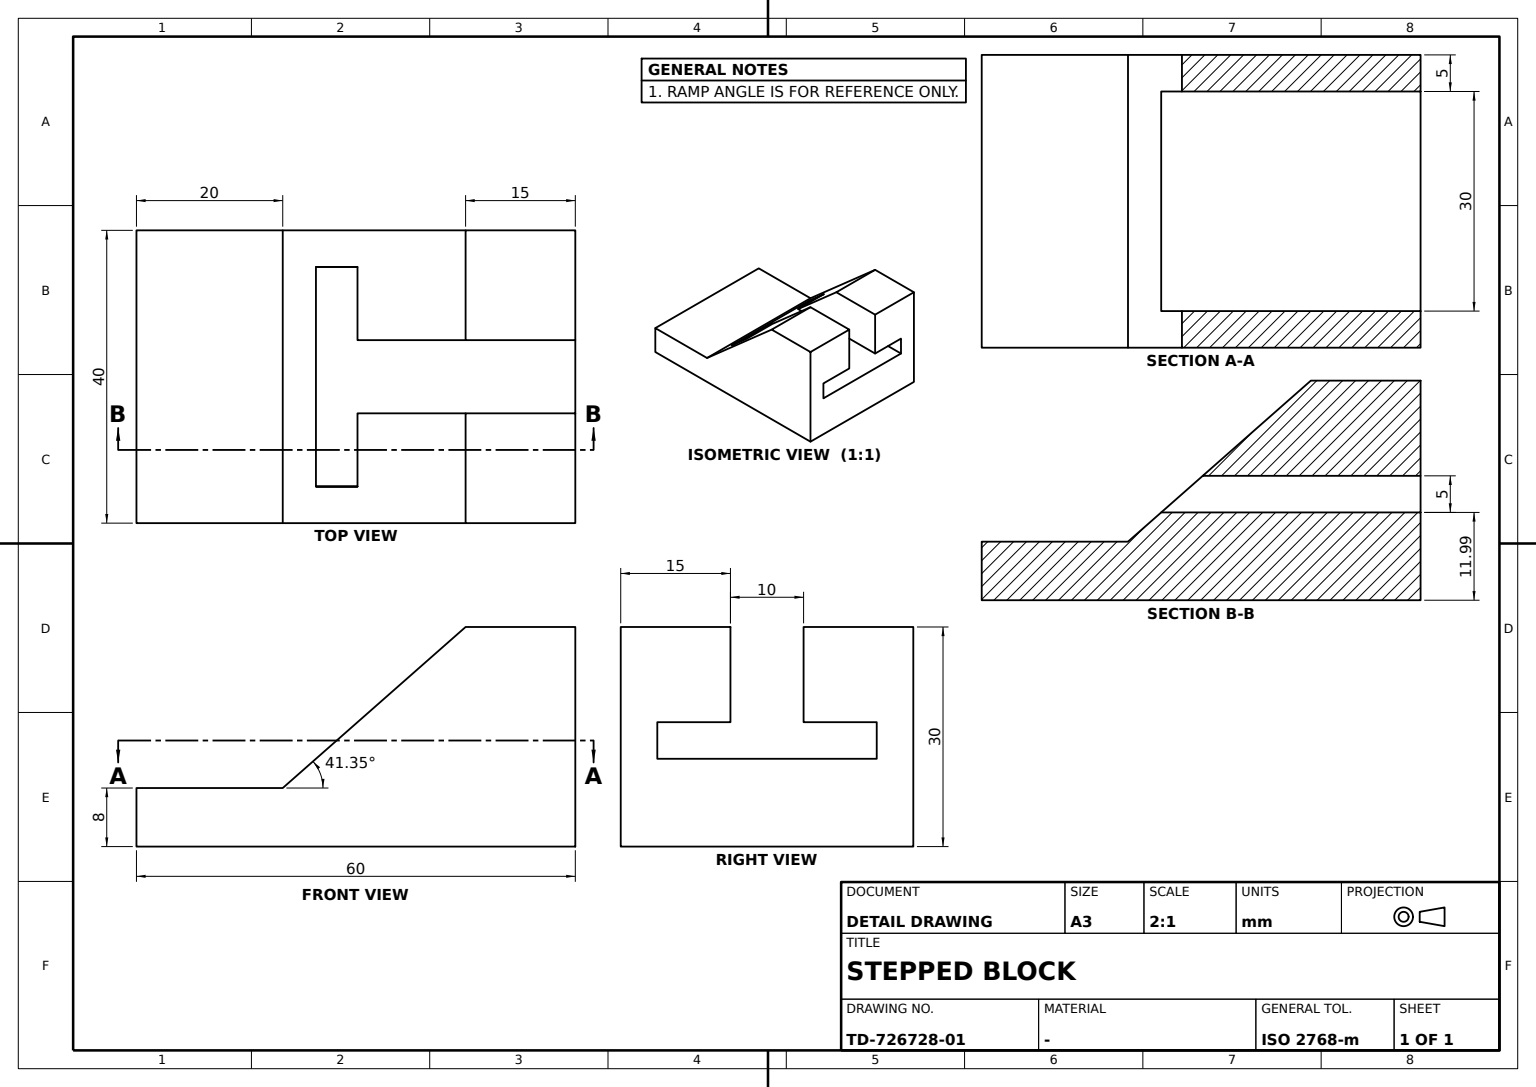
ISO-10303-21;
HEADER;
FILE_DESCRIPTION((''),'2;1');
FILE_NAME('','',(''),(''),'','','');
FILE_SCHEMA(('AUTOMOTIVE_DESIGN'));
ENDSEC;
DATA;
#1=APPLICATION_CONTEXT('');
#2=PRODUCT_CONTEXT('',#1,'mechanical');
#3=PRODUCT('','','',(#2));
#4=PRODUCT_DEFINITION_FORMATION('','',#3);
#5=PRODUCT_DEFINITION_CONTEXT('',#1,'design');
#6=PRODUCT_DEFINITION('','',#4,#5);
#7=PRODUCT_DEFINITION_SHAPE('','',#6);
#8=(LENGTH_UNIT()NAMED_UNIT(*)SI_UNIT(.MILLI.,.METRE.));
#9=(NAMED_UNIT(*)PLANE_ANGLE_UNIT()SI_UNIT($,.RADIAN.));
#10=(NAMED_UNIT(*)SI_UNIT($,.STERADIAN.)SOLID_ANGLE_UNIT());
#11=UNCERTAINTY_MEASURE_WITH_UNIT(LENGTH_MEASURE(0.005),#8,'distance_accuracy_value','');
#12=(GEOMETRIC_REPRESENTATION_CONTEXT(3)GLOBAL_UNCERTAINTY_ASSIGNED_CONTEXT((#11))GLOBAL_UNIT_ASSIGNED_CONTEXT((#8,#9,#10))REPRESENTATION_CONTEXT('',''));
#13=CARTESIAN_POINT('',(15.,-35.460872,11.994432));
#14=VERTEX_POINT('',#13);
#15=CARTESIAN_POINT('',(15.,-29.779054,16.994432));
#16=VERTEX_POINT('',#15);
#17=CARTESIAN_POINT('',(15.,-40.,8.));
#18=DIRECTION('',(0.,0.750713517,0.660627895));
#19=VECTOR('',#18,1000.);
#20=LINE('',#17,#19);
#21=EDGE_CURVE('',#14,#16,#20,.T.);
#22=ORIENTED_EDGE('',*,*,#21,.T.);
#23=CARTESIAN_POINT('',(15.,0.,16.994432));
#24=VERTEX_POINT('',#23);
#25=CARTESIAN_POINT('',(15.,-60.,16.994432));
#26=DIRECTION('',(0.,1.,0.));
#27=VECTOR('',#26,1000.);
#28=LINE('',#25,#27);
#29=EDGE_CURVE('',#16,#24,#28,.T.);
#30=ORIENTED_EDGE('',*,*,#29,.T.);
#31=CARTESIAN_POINT('',(15.,0.,11.994432));
#32=VERTEX_POINT('',#31);
#33=CARTESIAN_POINT('',(15.,0.,0.));
#34=DIRECTION('',(0.,0.,1.));
#35=VECTOR('',#34,1000.);
#36=LINE('',#33,#35);
#37=EDGE_CURVE('',#32,#24,#36,.T.);
#38=ORIENTED_EDGE('',*,*,#37,.F.);
#39=CARTESIAN_POINT('',(15.,-60.,11.994432));
#40=LINE('',#39,#27);
#41=EDGE_CURVE('',#14,#32,#40,.T.);
#42=ORIENTED_EDGE('',*,*,#41,.F.);
#43=EDGE_LOOP('',(#22,#30,#38,#42));
#44=FACE_BOUND('',#43,.T.);
#45=DIRECTION('',(-1.,0.,0.));
#46=AXIS2_PLACEMENT_3D('',#39,#45,#34);
#47=PLANE('',#46);
#48=ADVANCED_FACE('',(#44),#47,.T.);
#49=CARTESIAN_POINT('',(-20.,-60.,8.));
#50=VERTEX_POINT('',#49);
#51=CARTESIAN_POINT('',(-20.,-40.,8.));
#52=VERTEX_POINT('',#51);
#53=CARTESIAN_POINT('',(-20.,0.,8.));
#54=LINE('',#53,#27);
#55=EDGE_CURVE('',#50,#52,#54,.T.);
#56=ORIENTED_EDGE('',*,*,#55,.F.);
#57=CARTESIAN_POINT('',(20.,-60.,8.));
#58=VERTEX_POINT('',#57);
#59=CARTESIAN_POINT('',(0.,-60.,8.));
#60=DIRECTION('',(1.,0.,0.));
#61=VECTOR('',#60,1000.);
#62=LINE('',#59,#61);
#63=EDGE_CURVE('',#50,#58,#62,.T.);
#64=ORIENTED_EDGE('',*,*,#63,.T.);
#65=CARTESIAN_POINT('',(20.,-40.,8.));
#66=VERTEX_POINT('',#65);
#67=CARTESIAN_POINT('',(20.,0.,8.));
#68=LINE('',#67,#27);
#69=EDGE_CURVE('',#58,#66,#68,.T.);
#70=ORIENTED_EDGE('',*,*,#69,.T.);
#71=CARTESIAN_POINT('',(0.,-40.,8.));
#72=LINE('',#71,#61);
#73=EDGE_CURVE('',#52,#66,#72,.T.);
#74=ORIENTED_EDGE('',*,*,#73,.F.);
#75=EDGE_LOOP('',(#56,#64,#70,#74));
#76=FACE_BOUND('',#75,.T.);
#77=DIRECTION('',(0.,0.,-1.));
#78=AXIS2_PLACEMENT_3D('',#59,#77,#26);
#79=PLANE('',#78);
#80=ADVANCED_FACE('',(#76),#79,.F.);
#81=CARTESIAN_POINT('',(20.,0.,30.));
#82=VERTEX_POINT('',#81);
#83=CARTESIAN_POINT('',(20.,-15.,30.));
#84=VERTEX_POINT('',#83);
#85=DIRECTION('',(0.,-1.,0.));
#86=VECTOR('',#85,1000.);
#87=LINE('',#81,#86);
#88=EDGE_CURVE('',#82,#84,#87,.T.);
#89=ORIENTED_EDGE('',*,*,#88,.T.);
#90=CARTESIAN_POINT('',(20.,-21.424707,24.346258));
#91=LINE('',#90,#19);
#92=EDGE_CURVE('',#66,#84,#91,.T.);
#93=ORIENTED_EDGE('',*,*,#92,.F.);
#94=ORIENTED_EDGE('',*,*,#69,.F.);
#95=CARTESIAN_POINT('',(20.,-60.,0.));
#96=VERTEX_POINT('',#95);
#97=LINE('',#95,#35);
#98=EDGE_CURVE('',#96,#58,#97,.T.);
#99=ORIENTED_EDGE('',*,*,#98,.F.);
#100=CARTESIAN_POINT('',(20.,0.,0.));
#101=VERTEX_POINT('',#100);
#102=LINE('',#100,#86);
#103=EDGE_CURVE('',#101,#96,#102,.T.);
#104=ORIENTED_EDGE('',*,*,#103,.F.);
#105=LINE('',#100,#35);
#106=EDGE_CURVE('',#101,#82,#105,.T.);
#107=ORIENTED_EDGE('',*,*,#106,.T.);
#108=EDGE_LOOP('',(#89,#93,#94,#99,#104,#107));
#109=FACE_BOUND('',#108,.T.);
#110=AXIS2_PLACEMENT_3D('',#100,#60,#26);
#111=PLANE('',#110);
#112=ADVANCED_FACE('',(#109),#111,.T.);
#113=CARTESIAN_POINT('',(-5.,-29.779054,16.994432));
#114=VERTEX_POINT('',#113);
#115=CARTESIAN_POINT('',(-5.,0.,16.994432));
#116=VERTEX_POINT('',#115);
#117=CARTESIAN_POINT('',(-5.,-60.,16.994432));
#118=LINE('',#117,#27);
#119=EDGE_CURVE('',#114,#116,#118,.T.);
#120=ORIENTED_EDGE('',*,*,#119,.F.);
#121=CARTESIAN_POINT('',(-15.,-29.779054,16.994432));
#122=VERTEX_POINT('',#121);
#123=CARTESIAN_POINT('',(0.,-29.779054,16.994432));
#124=VECTOR('',#45,1000.);
#125=LINE('',#123,#124);
#126=EDGE_CURVE('',#114,#122,#125,.T.);
#127=ORIENTED_EDGE('',*,*,#126,.T.);
#128=CARTESIAN_POINT('',(-15.,0.,16.994432));
#129=VERTEX_POINT('',#128);
#130=CARTESIAN_POINT('',(-15.,-60.,16.994432));
#131=LINE('',#130,#27);
#132=EDGE_CURVE('',#122,#129,#131,.T.);
#133=ORIENTED_EDGE('',*,*,#132,.T.);
#134=CARTESIAN_POINT('',(0.,0.,16.994432));
#135=LINE('',#134,#124);
#136=EDGE_CURVE('',#116,#129,#135,.T.);
#137=ORIENTED_EDGE('',*,*,#136,.F.);
#138=EDGE_LOOP('',(#120,#127,#133,#137));
#139=FACE_BOUND('',#138,.T.);
#140=AXIS2_PLACEMENT_3D('',#25,#77,#45);
#141=PLANE('',#140);
#142=ADVANCED_FACE('',(#139),#141,.T.);
#143=CARTESIAN_POINT('',(5.,-29.779054,16.994432));
#144=VERTEX_POINT('',#143);
#145=CARTESIAN_POINT('',(5.,-15.,30.));
#146=VERTEX_POINT('',#145);
#147=CARTESIAN_POINT('',(5.,-40.,8.));
#148=LINE('',#147,#19);
#149=EDGE_CURVE('',#144,#146,#148,.T.);
#150=ORIENTED_EDGE('',*,*,#149,.F.);
#151=EDGE_CURVE('',#16,#144,#125,.T.);
#152=ORIENTED_EDGE('',*,*,#151,.F.);
#153=ORIENTED_EDGE('',*,*,#21,.F.);
#154=CARTESIAN_POINT('',(-15.,-35.460872,11.994432));
#155=VERTEX_POINT('',#154);
#156=CARTESIAN_POINT('',(0.,-35.460872,11.994432));
#157=LINE('',#156,#61);
#158=EDGE_CURVE('',#155,#14,#157,.T.);
#159=ORIENTED_EDGE('',*,*,#158,.F.);
#160=CARTESIAN_POINT('',(-15.,-40.,8.));
#161=DIRECTION('',(0.,-0.750713517,-0.660627895));
#162=VECTOR('',#161,1000.);
#163=LINE('',#160,#162);
#164=EDGE_CURVE('',#122,#155,#163,.T.);
#165=ORIENTED_EDGE('',*,*,#164,.F.);
#166=ORIENTED_EDGE('',*,*,#126,.F.);
#167=CARTESIAN_POINT('',(-5.,-15.,30.));
#168=VERTEX_POINT('',#167);
#169=CARTESIAN_POINT('',(-5.,-40.223483,7.803335));
#170=LINE('',#169,#19);
#171=EDGE_CURVE('',#114,#168,#170,.T.);
#172=ORIENTED_EDGE('',*,*,#171,.T.);
#173=CARTESIAN_POINT('',(-20.,-15.,30.));
#174=VERTEX_POINT('',#173);
#175=CARTESIAN_POINT('',(0.,-15.,30.));
#176=LINE('',#175,#61);
#177=EDGE_CURVE('',#174,#168,#176,.T.);
#178=ORIENTED_EDGE('',*,*,#177,.F.);
#179=CARTESIAN_POINT('',(-20.,-21.424707,24.346258));
#180=LINE('',#179,#19);
#181=EDGE_CURVE('',#52,#174,#180,.T.);
#182=ORIENTED_EDGE('',*,*,#181,.F.);
#183=ORIENTED_EDGE('',*,*,#73,.T.);
#184=ORIENTED_EDGE('',*,*,#92,.T.);
#185=EDGE_CURVE('',#146,#84,#176,.T.);
#186=ORIENTED_EDGE('',*,*,#185,.F.);
#187=EDGE_LOOP('',(#150,#152,#153,#159,#165,#166,#172,#178,#182,#183,#184,#186));
#188=FACE_BOUND('',#187,.T.);
#189=DIRECTION('',(0.,0.660627895,-0.750713517));
#190=AXIS2_PLACEMENT_3D('',#71,#189,#18);
#191=PLANE('',#190);
#192=ADVANCED_FACE('',(#188),#191,.F.);
#193=CARTESIAN_POINT('',(5.,0.,30.));
#194=VERTEX_POINT('',#193);
#195=LINE('',#193,#86);
#196=EDGE_CURVE('',#194,#146,#195,.T.);
#197=ORIENTED_EDGE('',*,*,#196,.F.);
#198=CARTESIAN_POINT('',(5.,0.,16.994432));
#199=VERTEX_POINT('',#198);
#200=CARTESIAN_POINT('',(5.,0.,0.));
#201=LINE('',#200,#35);
#202=EDGE_CURVE('',#199,#194,#201,.T.);
#203=ORIENTED_EDGE('',*,*,#202,.F.);
#204=CARTESIAN_POINT('',(5.,-60.,16.994432));
#205=LINE('',#204,#27);
#206=EDGE_CURVE('',#144,#199,#205,.T.);
#207=ORIENTED_EDGE('',*,*,#206,.F.);
#208=ORIENTED_EDGE('',*,*,#149,.T.);
#209=EDGE_LOOP('',(#197,#203,#207,#208));
#210=FACE_BOUND('',#209,.T.);
#211=AXIS2_PLACEMENT_3D('',#204,#45,#34);
#212=PLANE('',#211);
#213=ADVANCED_FACE('',(#210),#212,.T.);
#214=CARTESIAN_POINT('',(-5.,0.,30.));
#215=VERTEX_POINT('',#214);
#216=CARTESIAN_POINT('',(-5.,0.,30.276649));
#217=LINE('',#216,#35);
#218=EDGE_CURVE('',#116,#215,#217,.T.);
#219=ORIENTED_EDGE('',*,*,#218,.T.);
#220=CARTESIAN_POINT('',(-5.,-60.,30.));
#221=LINE('',#220,#86);
#222=EDGE_CURVE('',#215,#168,#221,.T.);
#223=ORIENTED_EDGE('',*,*,#222,.T.);
#224=ORIENTED_EDGE('',*,*,#171,.F.);
#225=ORIENTED_EDGE('',*,*,#119,.T.);
#226=EDGE_LOOP('',(#219,#223,#224,#225));
#227=FACE_BOUND('',#226,.T.);
#228=CARTESIAN_POINT('',(-5.,-60.,30.276649));
#229=AXIS2_PLACEMENT_3D('',#228,#60,#77);
#230=PLANE('',#229);
#231=ADVANCED_FACE('',(#227),#230,.T.);
#232=CARTESIAN_POINT('',(-20.,-60.,0.));
#233=VERTEX_POINT('',#232);
#234=CARTESIAN_POINT('',(0.,-60.,0.));
#235=LINE('',#234,#61);
#236=EDGE_CURVE('',#233,#96,#235,.T.);
#237=ORIENTED_EDGE('',*,*,#236,.F.);
#238=CARTESIAN_POINT('',(-20.,0.,0.));
#239=VERTEX_POINT('',#238);
#240=LINE('',#238,#86);
#241=EDGE_CURVE('',#239,#233,#240,.T.);
#242=ORIENTED_EDGE('',*,*,#241,.F.);
#243=CARTESIAN_POINT('',(0.,0.,0.));
#244=LINE('',#243,#61);
#245=EDGE_CURVE('',#239,#101,#244,.T.);
#246=ORIENTED_EDGE('',*,*,#245,.T.);
#247=ORIENTED_EDGE('',*,*,#103,.T.);
#248=EDGE_LOOP('',(#237,#242,#246,#247));
#249=FACE_BOUND('',#248,.T.);
#250=AXIS2_PLACEMENT_3D('',#243,#34,#85);
#251=PLANE('',#250);
#252=ADVANCED_FACE('',(#249),#251,.F.);
#253=CARTESIAN_POINT('',(-20.,0.,30.));
#254=VERTEX_POINT('',#253);
#255=LINE('',#253,#86);
#256=EDGE_CURVE('',#254,#174,#255,.T.);
#257=ORIENTED_EDGE('',*,*,#256,.T.);
#258=ORIENTED_EDGE('',*,*,#177,.T.);
#259=ORIENTED_EDGE('',*,*,#222,.F.);
#260=CARTESIAN_POINT('',(0.,0.,30.));
#261=LINE('',#260,#61);
#262=EDGE_CURVE('',#254,#215,#261,.T.);
#263=ORIENTED_EDGE('',*,*,#262,.F.);
#264=EDGE_LOOP('',(#257,#258,#259,#263));
#265=FACE_BOUND('',#264,.T.);
#266=AXIS2_PLACEMENT_3D('',#260,#34,#85);
#267=PLANE('',#266);
#268=ADVANCED_FACE('',(#265),#267,.T.);
#269=ORIENTED_EDGE('',*,*,#164,.T.);
#270=CARTESIAN_POINT('',(-15.,0.,11.994432));
#271=VERTEX_POINT('',#270);
#272=CARTESIAN_POINT('',(-15.,-60.,11.994432));
#273=LINE('',#272,#27);
#274=EDGE_CURVE('',#155,#271,#273,.T.);
#275=ORIENTED_EDGE('',*,*,#274,.T.);
#276=CARTESIAN_POINT('',(-15.,0.,0.));
#277=VECTOR('',#77,1000.);
#278=LINE('',#276,#277);
#279=EDGE_CURVE('',#129,#271,#278,.T.);
#280=ORIENTED_EDGE('',*,*,#279,.F.);
#281=ORIENTED_EDGE('',*,*,#132,.F.);
#282=EDGE_LOOP('',(#269,#275,#280,#281));
#283=FACE_BOUND('',#282,.T.);
#284=AXIS2_PLACEMENT_3D('',#130,#60,#77);
#285=PLANE('',#284);
#286=ADVANCED_FACE('',(#283),#285,.T.);
#287=EDGE_CURVE('',#24,#199,#135,.T.);
#288=ORIENTED_EDGE('',*,*,#287,.F.);
#289=ORIENTED_EDGE('',*,*,#29,.F.);
#290=ORIENTED_EDGE('',*,*,#151,.T.);
#291=ORIENTED_EDGE('',*,*,#206,.T.);
#292=EDGE_LOOP('',(#288,#289,#290,#291));
#293=FACE_BOUND('',#292,.T.);
#294=ADVANCED_FACE('',(#293),#141,.T.);
#295=ORIENTED_EDGE('',*,*,#158,.T.);
#296=ORIENTED_EDGE('',*,*,#41,.T.);
#297=CARTESIAN_POINT('',(0.,0.,11.994432));
#298=LINE('',#297,#61);
#299=EDGE_CURVE('',#271,#32,#298,.T.);
#300=ORIENTED_EDGE('',*,*,#299,.F.);
#301=ORIENTED_EDGE('',*,*,#274,.F.);
#302=EDGE_LOOP('',(#295,#296,#300,#301));
#303=FACE_BOUND('',#302,.T.);
#304=AXIS2_PLACEMENT_3D('',#272,#34,#60);
#305=PLANE('',#304);
#306=ADVANCED_FACE('',(#303),#305,.T.);
#307=ORIENTED_EDGE('',*,*,#299,.T.);
#308=ORIENTED_EDGE('',*,*,#37,.T.);
#309=ORIENTED_EDGE('',*,*,#287,.T.);
#310=ORIENTED_EDGE('',*,*,#202,.T.);
#311=EDGE_CURVE('',#194,#82,#261,.T.);
#312=ORIENTED_EDGE('',*,*,#311,.T.);
#313=ORIENTED_EDGE('',*,*,#106,.F.);
#314=ORIENTED_EDGE('',*,*,#245,.F.);
#315=LINE('',#238,#35);
#316=EDGE_CURVE('',#239,#254,#315,.T.);
#317=ORIENTED_EDGE('',*,*,#316,.T.);
#318=ORIENTED_EDGE('',*,*,#262,.T.);
#319=ORIENTED_EDGE('',*,*,#218,.F.);
#320=ORIENTED_EDGE('',*,*,#136,.T.);
#321=ORIENTED_EDGE('',*,*,#279,.T.);
#322=EDGE_LOOP('',(#307,#308,#309,#310,#312,#313,#314,#317,#318,#319,#320,#321));
#323=FACE_BOUND('',#322,.T.);
#324=AXIS2_PLACEMENT_3D('',#243,#26,#34);
#325=PLANE('',#324);
#326=ADVANCED_FACE('',(#323),#325,.T.);
#327=LINE('',#232,#35);
#328=EDGE_CURVE('',#233,#50,#327,.T.);
#329=ORIENTED_EDGE('',*,*,#328,.T.);
#330=ORIENTED_EDGE('',*,*,#55,.T.);
#331=ORIENTED_EDGE('',*,*,#181,.T.);
#332=ORIENTED_EDGE('',*,*,#256,.F.);
#333=ORIENTED_EDGE('',*,*,#316,.F.);
#334=ORIENTED_EDGE('',*,*,#241,.T.);
#335=EDGE_LOOP('',(#329,#330,#331,#332,#333,#334));
#336=FACE_BOUND('',#335,.T.);
#337=AXIS2_PLACEMENT_3D('',#238,#60,#26);
#338=PLANE('',#337);
#339=ADVANCED_FACE('',(#336),#338,.F.);
#340=ORIENTED_EDGE('',*,*,#311,.F.);
#341=ORIENTED_EDGE('',*,*,#196,.T.);
#342=ORIENTED_EDGE('',*,*,#185,.T.);
#343=ORIENTED_EDGE('',*,*,#88,.F.);
#344=EDGE_LOOP('',(#340,#341,#342,#343));
#345=FACE_BOUND('',#344,.T.);
#346=ADVANCED_FACE('',(#345),#267,.T.);
#347=ORIENTED_EDGE('',*,*,#98,.T.);
#348=ORIENTED_EDGE('',*,*,#63,.F.);
#349=ORIENTED_EDGE('',*,*,#328,.F.);
#350=ORIENTED_EDGE('',*,*,#236,.T.);
#351=EDGE_LOOP('',(#347,#348,#349,#350));
#352=FACE_BOUND('',#351,.T.);
#353=AXIS2_PLACEMENT_3D('',#234,#26,#34);
#354=PLANE('',#353);
#355=ADVANCED_FACE('',(#352),#354,.F.);
#356=CLOSED_SHELL('',(#48,#80,#112,#142,#192,#213,#231,#252,#268,#286,#294,#306,#326,#339,#346,#355));
#357=MANIFOLD_SOLID_BREP('',#356);
#358=ADVANCED_BREP_SHAPE_REPRESENTATION('',(#357),#12);
#359=SHAPE_DEFINITION_REPRESENTATION(#7,#358);
ENDSEC;
END-ISO-10303-21;
